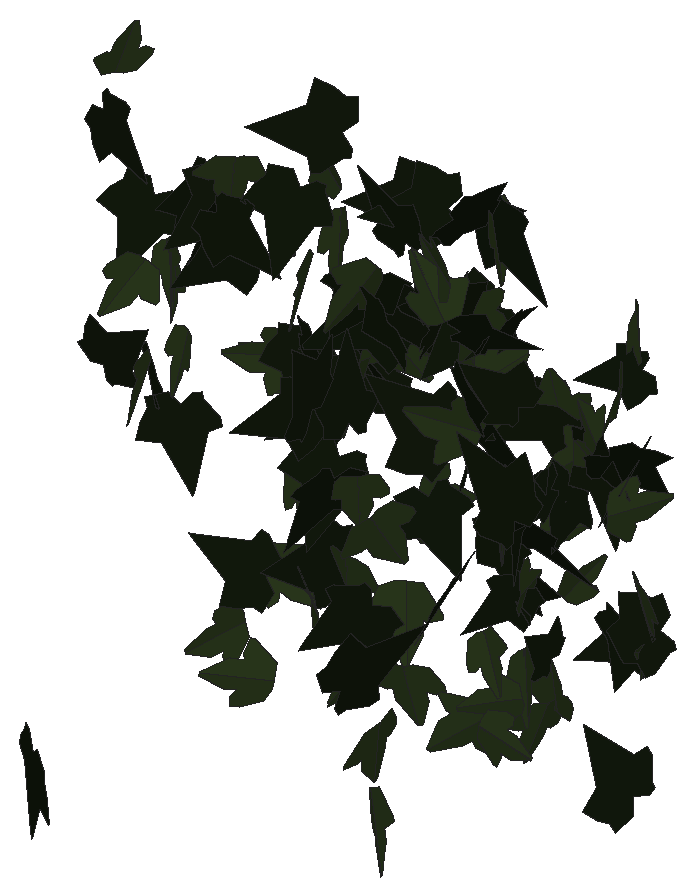
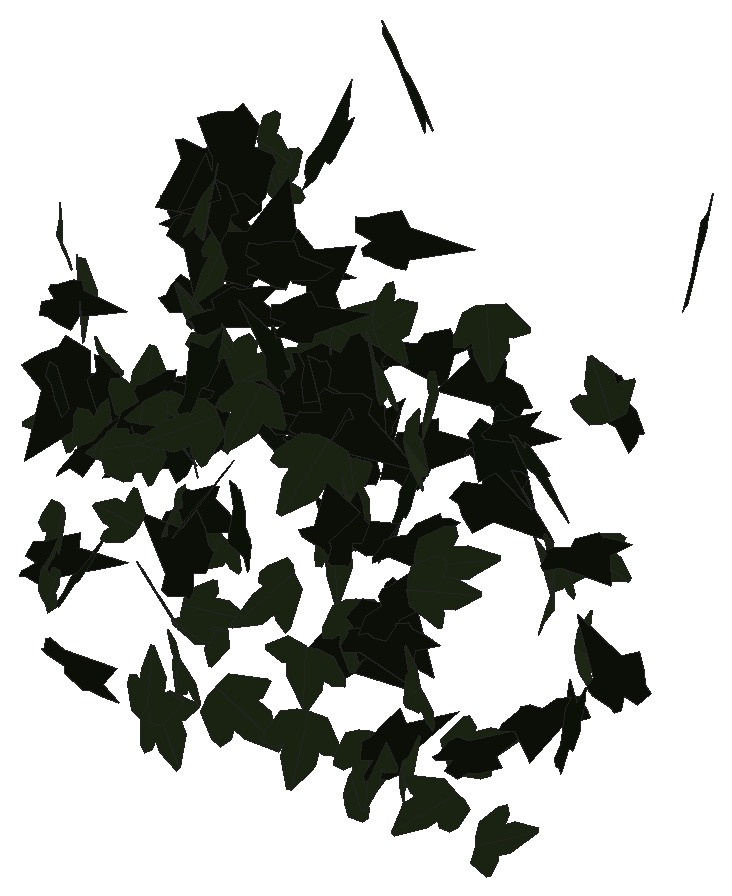
# SketchUp Ruby script. Lengths in inches.
U = 1.inch
M = Sketchup.active_model
def pt(a) = Geom::Point3d.new(a.map { |v| v * U })
def face(e, loops, mat)
  f = e.add_face(loops[0].map { |a| pt(a) })
  loops[1..].each { |l| e.add_face(l.map { |a| pt(a) }).erase! }
  f.material = f.back_material = mat if mat
  f
end
# faces: each face lists its corners as indices into pts; further lists are holes
def faces(e, pts, list, mat = nil) = list.each { |f| face(e, (f[0].is_a?(Array) ? f : [f]).map { |l| l.map { |i| pts[i] } }, mat) }
# xy, xz, yz: faces in a plane at the given z, y or x. An outline is a flat list of corners, or four numbers for a rectangle; further outlines are holes
def ring(l) = l.size == 4 ? [[l[0], l[1]], [l[2], l[1]], [l[2], l[3]], [l[0], l[3]]] : l.each_slice(2).to_a
def flat(e, list, mat, &to3) = list.each { |f| face(e, (f[0].is_a?(Array) ? f : [f]).map { |l| ring(l).map { |u, v| to3.(u, v) } }, mat) }
def xy(e, z, list, mat = nil) = flat(e, list, mat) { |x, y| [x, y, z] }
def xz(e, y, list, mat = nil) = flat(e, list, mat) { |x, z| [x, y, z] }
def yz(e, x, list, mat = nil) = flat(e, list, mat) { |y, z| [x, y, z] }
def lines(e, pts, list) = list.each { |a, b| e.add_line(pt(pts[a]), pt(pts[b])) }
# prism: a flat outline (further loops are holes) pulled along v
def prism(e, loops, v, mat = nil)
  f = face(e, loops, mat); d = Geom::Vector3d.new(v.map { |x| x * U })
  f.pushpull(f.normal.samedirection?(d) ? d.length : -d.length)
end
def box(e, o, s, mat = nil) = prism(e, [[o, [o[0] + s[0], o[1], o[2]], [o[0] + s[0], o[1] + s[1], o[2]], [o[0], o[1] + s[1], o[2]]]], [0, 0, s[2]], mat)
def at(x, y, z, deg = 0) = Geom::Transformation.translation(pt([x, y, z])) * Geom::Transformation.rotation(ORIGIN, Z_AXIS, deg.degrees)
def axes(o, x, y, z) = Geom::Transformation.new([*x, 0, *y, 0, *z, 0, *pt(o).to_a, 1])
def part(name) = M.definitions.add(name)
# library, detail: a bought-in or finely detailed component or shape, given as its bounding box
def library(name, o, s) = part(name).tap { |d| box(d.entities, o, s) }
def detail(e, o, s) = box(e.add_group.entities, o, s)
def put(e, d, t, mat = nil) = e.add_instance(d, t).tap { |i| i.material = mat if mat }
def group(e, t, mat = nil) = e.add_group.tap { |g| g.transformation = t; g.material = mat if mat }.entities
root = M.entities
M.materials.add("efeu1").color = [18, 25, 13]
M.materials.add("efeu2").color = [43, 57, 29]
c1 = part("ivyleaf_9")
p = [[1.54,2.16,1.25],[1.36,2.04,1.19],[-0.21,0.99,0.68],[-0.71,1.11,0.82],[-0.85,0.86,0.67],[-0.8,0.17,0.21],
  [-0.9,-0.01,0.1],[-0.67,-0.16,-0.02],[-0.08,-0.08,-0.05],[-0.03,-0.6,-0.4],[0.65,-0.88,-0.66],[0.83,-0.6,-0.49],
  [1.29,-0.42,-0.43],[1.8125,-0.07,-0.26],[1.21,0.44,0.15]]
faces(c1.entities,p,[[0,1,2,3,4,5,6,7,8,9,10,11,12,13,14]],"efeu1")
c2 = part("ivyleaf_10")
p = [[0,0.5,-0.03],[-0.0625,2.02,-0.43],[-0.19,2.01,-0.46],[-0.54,1.05,-0.29],[-0.52,0.625,-0.18],[-0.83,0.76,-0.28],
  [-1.16,0.64,-0.33],[-1.15,0.33,-0.24],[-0.77,-0.39,0.02],[-0.3,-0.51,0.16],[0.04,-0.48,0.23],[-0.02,2.01,-0.4375],
  [-0.06,2.01,-0.43],[0.04,-0.49,0.23],[0.67,-0.49,0.14],[1.38,0.36,-0.2],[1.375,0.51,-0.24],[0.81,0.65,-0.19],
  [0.62,0.59,-0.15],[0.6,1.09,-0.28],[0.5,1.23,-0.31]]
faces(c2.entities,p,[[0,1,2,3,4,5,6,7,8,9,10],[11,12,0,13,14,15,16,17,18,19,20]],"efeu2")
put(root,c1,axes([576.6875,99.81,193.13],[0.37598,-0.23293,-1.38227],[1.25923,-0.57264,0.43901],[-0.61586,-1.31306,0.05375]))
put(root,c2,axes([583.77,110.99,188.68],[-0.42455,1.04749,-0.55022],[0.21582,-0.5062,-1.13022],[-1.16335,-0.47618,-0.00888]))
put(root,c1,axes([580.52,111.29,204.13],[-0.34881,0.80332,1.20672],[-0.45266,1.11874,-0.8756],[-1.37717,-0.57118,-0.01783]))
put(root,c1,axes([579.57,114.39,190.66],[0.12861,0.13692,1.33146],[1.00054,0.87864,-0.187],[-0.88907,1.00862,-0.01785]))
put(root,c2,axes([579.82,116.01,188.12],[-0.00624,-1.2313,-0.24566],[0.00097,0.24566,-1.23131],[1.25556,-0.00631,-0.00027]))
put(root,c1,axes([578.77,117.87,204.16],[0.79532,-0.66978,-0.56365],[0.43288,-0.361,1.03978],[-0.76087,-0.90549,0.00238]))
put(root,c2,axes([579.15,116.83,196.28],[-0.58735,-0.9171,-0.59938],[0.3209,0.50625,-1.08906],[1.04755,-0.66929,-0.00245]))
put(root,c1,axes([585.18,117.21,198.54],[-0.07861,0.19519,1.39451],[-0.99968,0.97588,-0.19295],[-0.99166,-0.99925,0.08396]))
put(root,c1,axes([581.57,118.33,194.09],[-0.6526,0.81064,-0.47546],[0.30079,-0.36823,-1.04068],[-0.89035,-0.71858,-0.00308]))
put(root,c1,axes([579.63,119.36,196.36],[-0.04157,-0.87284,-0.66564],[0.05238,0.66378,-0.87368],[1.09644,-0.0648,0.0165]))
put(root,c2,axes([579.4,120.19,204.02],[0.9037,0.26235,0.6247],[-0.60418,-0.15932,0.94092],[0.30667,-1.08699,0.01286]))
put(root,c2,axes([570.34,120.92,184.91],[0.0741,0.27954,1.0388],[-0.499,-0.91353,0.28142],[0.95302,-0.50005,0.06658]))
put(root,c1,axes([580.01,120.97,200.04],[0.13894,-0.23607,0.99025],[0.46186,-0.87604,-0.27364],[0.90721,0.48214,-0.01235]))
put(root,c2,axes([579.59,120.0625,205.41],[-0.16108,0.12198,-1.11142],[-0.80563,0.76597,0.20083],[0.7753,0.82128,-0.02223]))
put(root,c1,axes([572.14,121.73,196.54],[-0.13488,-0.4355,-0.98711],[-0.03088,-0.99283,0.44225],[-1.07847,0.08289,0.11079]))
put(root,c2,axes([580.61,121.3125,189.78],[0.76357,-0.05982,0.61897],[0.61628,-0.05814,-0.76587],[0.08306,0.98122,-0.00765]))
put(root,c2,axes([580.89,121.37,186.2],[-0.24339,0.00696,-0.94198],[0.90391,-0.27215,-0.23557],[-0.26517,-0.93408,0.06162]))
put(root,c1,axes([579.82,121.11,202.6875],[0.72154,-0.01298,0.70616],[0.70553,0.05985,-0.71979],[-0.03261,1.00782,0.05184]))
put(root,c2,axes([581.09,122.14,187.29],[-0.10062,-0.13892,0.92067],[-0.59928,-0.69906,-0.17098],[0.7126,-0.60751,-0.01378]))
put(root,c2,axes([580.64,122.12,194.78],[-0.28531,0.51157,-0.73913],[0.34535,-0.65356,-0.58567],[-0.82991,-0.44785,0.01039]))
put(root,c1,axes([574.33,122.4,188.66],[0.0712,0.10786,-1.10788],[-0.49243,-0.99255,-0.12828],[-0.99827,0.4973,-0.01574]))
put(root,c2,axes([578.68,122.66,197.54],[-0.36943,-0.22943,-1.12963],[-0.96314,-0.59027,0.43487],[-0.63329,1.03156,-0.0024]))
put(root,c1,axes([581.09,122.76,191.55],[-0.03661,0.00225,-0.90716],[0.02991,-0.9074,-0.00345],[-0.90667,-0.03002,0.03652]))
put(root,c1,axes([577.67,122.625,202.2],[0.79036,0.26559,0.76895],[-0.7268,-0.25115,0.83377],[0.3655,-1.07372,-0.00482]))
put(root,c1,axes([573.625,122.07,196.45],[-0.43939,-0.68038,0.79048],[0.4057,0.67871,0.80969],[-0.96082,0.59772,-0.0196]))
put(root,c1,axes([581,122.63,199.39],[-0.03845,0.13449,0.9198],[-0.92952,0.00545,-0.03965],[-0.01112,-0.92059,0.13414]))
put(root,c1,axes([581.01,122.82,194.7],[-0.37558,-0.01683,-0.8276],[0.81422,-0.17129,-0.36603],[-0.14917,-0.89255,0.08584]))
put(root,c1,axes([577.45,122.69,196.76],[-1.01125,-0.48445,-0.67672],[-0.59369,-0.3264,1.12083],[-0.58325,1.17219,0.03242]))
put(root,c1,axes([581.4,122.35,194.54],[1.24264,-0.12436,0.23053],[0.22958,-0.02103,-1.24885],[0.12611,1.26367,0.00191]))
put(root,c1,axes([580.64,122.2,202.56],[0.05643,0.9385,0.17844],[0.00155,0.17866,-0.94015],[-0.95531,0.05572,0.00902]))
put(root,c2,axes([573.26,123.5,201.58],[-0.07924,-0.77106,0.88087],[-0.01064,-0.88238,-0.77333],[1.17062,-0.06022,0.0526]))
put(root,c2,axes([578.72,123.35,185.03],[-0.57796,-0.45111,0.95395],[-0.76465,-0.5705,-0.73306],[0.7272,-0.95842,-0.01265]))
put(root,c2,axes([579.44,122.43,202.56],[-0.10194,-0.82834,-0.8697],[0.27644,0.83321,-0.82599],[1.16881,-0.26931,0.11951]))
put(root,c2,axes([564.78,123.42,195.9375],[0.84954,-0.58492,0.13821],[0.11518,-0.07643,-1.03142],[0.58988,0.85731,0.00235]))
put(root,c1,axes([578.58,122.27,206.5],[0.5658,0.85095,0.73106],[0.39266,0.61678,-1.02181],[-1.0509,0.6886,0.01181]))
put(root,c1,axes([566.67,123.21,202.02],[0.0796,-0.21733,-1.11977],[0.93687,0.65277,-0.06009],[0.65068,-0.91329,0.22351]))
put(root,c1,axes([579.47,123.6,193.05],[0.53696,-1.07695,-0.0969],[-0.04223,0.08722,-1.20339],[1.08048,0.53862,0.00112]))
put(root,c2,axes([567.19,123.43,204.2],[-0.74535,-0.74022,0.08376],[-0.05925,-0.05921,-1.05046],[0.74258,-0.7477,0.00026]))
put(root,c2,axes([581.22,122.78,191.65],[-0.00272,-0.15871,-0.88095],[-0.07317,0.87805,-0.15796],[0.89214,0.07153,-0.01564]))
put(root,c1,axes([581.78,123.63,195.65],[-0.80952,0.29608,-0.1704],[0.15255,-0.07885,-0.8617],[-0.30566,-0.82349,0.02124]))
put(root,c2,axes([578.99,123.64,199.4],[0.73402,-0.27168,-0.86308],[0.83233,-0.23316,0.78126],[-0.35489,-1.10875,0.04719]))
put(root,c2,axes([566.47,124.34,184.18],[0.11187,0.15716,-1.04889],[-0.49494,-0.92508,-0.1914],[-0.93803,0.50685,-0.0241]))
put(root,c1,axes([578.38,123.94,197.02],[0.52187,-0.01064,-1.13102],[1.1276,0.10229,0.51933],[0.08845,-1.2414,0.05249]))
put(root,c2,axes([572.11,124.55,184.32],[0.00471,-0.14446,1.06579],[0.38185,-0.99615,-0.13671],[1.00547,0.37899,0.04692]))
put(root,c1,axes([567.87,124.27,186.92],[-0.52827,-0.84373,-0.40503],[-0.18535,-0.36157,0.99495],[-0.91738,0.55892,0.03221]))
put(root,c2,axes([562.1,124.5,193.34],[0.34739,-0.49754,0.88006],[0.50068,-0.72376,-0.60681],[0.87827,0.60939,-0.00217]))
put(root,c1,axes([579,123.96,205.91],[-0.17813,-0.08069,-1.29109],[1.20324,0.46823,-0.19528],[0.47502,-1.21631,0.01048]))
put(root,c1,axes([578.04,124.74,201.43],[-0.77449,-0.87377,0.45369],[-0.28368,-0.3547,-1.16741],[0.94278,-0.82453,0.02143]))
put(root,c2,axes([575.05,123.77,185.45],[-1.06568,-0.35712,-0.10063],[0.09572,0.03107,-1.12392],[0.35846,-1.06997,0.00095]))
put(root,c2,axes([574.7,123.97,188.46],[1.17891,0.23405,0.24291],[0.23853,0.04596,-1.20191],[-0.23851,1.20279,-0.00134]))
put(root,c1,axes([585.55,123.71,184.18],[-1.03675,-0.16771,-0.55972],[-0.55273,-0.08818,1.05022],[-0.18948,1.17488,-0.00107]))
put(root,c1,axes([571.08,124.34,191.92],[-0.17026,0.68314,-0.9242],[0.17731,-0.90749,-0.70345],[-1.13551,-0.24413,0.02873]))
put(root,c1,axes([560.51,124.23,203.73],[-0.00376,-0.1984,-1.09862],[1.06849,0.31772,-0.06103],[0.32351,-1.05168,0.18881]))
put(root,c1,axes([581.8,123.66,188.63],[-0.35075,0.51036,0.58361],[-0.33715,0.47641,-0.61924],[-0.69814,-0.48648,0.00583]))
put(root,c1,axes([572.98,124.18,201.08],[0.31311,0.62899,-0.95138],[-0.43056,-0.84839,-0.7026],[-1.05611,0.53235,0.00438]))
put(root,c2,axes([561.72,124.5625,197.375],[0.50217,0.5619,-0.68683],[-0.45573,-0.51386,-0.7536],[-0.76143,0.67813,-0.00193]))
put(root,c1,axes([571.125,124.59,206.5],[-0.7001,-0.05021,0.93375],[-0.92954,-0.08969,-0.70176],[0.10185,-1.16361,0.0138]))
put(root,c1,axes([581.73,124.95,195.07],[-0.07557,-0.90683,0.49811],[0.00475,-0.49973,-0.90906],[1.03461,-0.06394,0.04056]))
put(root,c2,axes([581.81,123.64,194],[-0.06949,-0.14341,-0.85498],[0.47056,0.71414,-0.15803],[0.72811,-0.47522,0.02053]))
put(root,c1,axes([574.51,124.16,203.42],[0.25263,-0.24003,1.001],[-0.7621,0.64925,0.34802],[-0.69197,-0.80268,-0.01784]))
put(root,c1,axes([569.05,124.85,203.19],[-0.62128,-0.96049,-0.15125],[0.0837,0.126,-1.14391],[0.96872,-0.62689,0.00183]))
put(root,c2,axes([578.71,124.44,205.7],[-0.32403,1.14319,-0.35051],[0.08306,-0.34075,-1.18816],[-1.19283,-0.33427,0.01248]))
put(root,c1,axes([575.75,124.0625,199.625],[-0.24948,0.97999,0.35571],[0.06059,-0.3515,1.0109],[1.04079,0.25537,0.02641]))
put(root,c1,axes([579.23,124.76,190.67],[0.30137,-0.30425,1.06123],[0.73438,-0.76612,-0.42819],[0.8243,0.79378,-0.00651]))
put(root,c2,axes([569.5,125,186],[-0.42874,0.09254,1.03856],[0.8937,-0.54581,0.41757],[0.53708,0.98209,0.13421]))
put(root,c2,axes([571.96,124.93,196.5625],[0.51208,-1.05709,0.37701],[0.17278,-0.33521,-1.17456],[1.10893,0.54037,0.00891]))
put(root,c2,axes([579.43,124.99,186.9],[0.81416,-0.35343,0.68704],[0.63444,-0.26378,-0.88753],[0.44093,1.03214,0.00844]))
put(root,c2,axes([584.4,124.36,200.44],[0.36155,-0.89247,-0.6503],[-0.22896,0.60881,-0.96283],[1.08026,0.42774,0.01358]))
put(root,c1,axes([572.9,125.22,199.24],[-0.02417,-0.06681,-1.27613],[-0.71896,-1.05448,0.06883],[-1.05644,0.71915,-0.01764]))
put(root,c2,axes([582.32,124.375,191.3],[-0.07325,-0.56841,0.60889],[0.06378,0.60561,0.57302],[-0.83052,0.09664,-0.0097]))
put(root,c1,axes([569.61,124.54,197.33],[0.73917,-0.3417,-0.62969],[-0.56379,0.28083,-0.8142],[0.44206,0.92953,0.01451]))
put(root,c1,axes([565.1875,125.74,201.1875],[-0.65175,-0.72254,0.59603],[-0.34064,-0.49356,-0.9708],[0.87252,-0.73241,0.06621]))
put(root,c1,axes([559.92,125.01,192.72],[-0.25218,0.04865,1.02424],[0.82065,-0.62281,0.23164],[0.61478,0.85133,0.11093]))
put(root,c2,axes([570.45,125.35,202.03],[0.88966,-0.48685,0.6537],[0.57213,-0.31622,-1.01416],[0.58053,1.05775,-0.00231]))
put(root,c2,axes([568.81,125.57,199.54],[0.53773,-0.67256,0.75229],[0.44877,-0.60411,-0.86086],[0.90381,0.7001,-0.02014]))
put(root,c1,axes([575.44,125.4375,204.45],[-0.77912,-0.09995,0.76812],[-0.7532,-0.15652,-0.78436],[0.18079,-1.08284,0.04247]))
put(root,c1,axes([573.13,124.91,200.1],[-0.00657,-0.0431,-1.13577],[0.96097,0.6063,-0.02857],[0.60694,-0.96042,0.03294]))
put(root,c2,axes([571.7,125.08,191.68],[-0.686,-0.72851,-0.02067],[0.02102,0.0086,-1.00062],[0.7285,-0.68626,0.00941]))
put(root,c1,axes([583.5,125.88,189.15],[0.03751,-0.82037,0.70868],[0.13206,-0.70037,-0.81773],[1.07601,0.11455,0.07565]))
put(root,c2,axes([580.0625,125.41,184.92],[-0.17895,-1.02248,0.25342],[-0.04918,-0.24866,-1.03801],[1.05227,-0.18551,-0.00542]))
put(root,c1,axes([584.5,125.375,196.99],[-0.6836,0.58659,-0.51199],[0.37107,-0.35352,-0.90047],[-0.68449,-0.77747,0.02316]))
put(root,c2,axes([567.77,125.72,195.43],[-0.01935,-0.00566,-1.13432],[-1.02381,-0.48838,0.0199],[-0.4884,1.02399,0.00322]))
put(root,c1,axes([580.33,126.1,197.55],[0.02923,-0.44999,-0.98319],[0.07057,-0.98066,0.45092],[-1.07897,-0.07633,0.00286]))
put(root,c1,axes([565.28,125.39,201.4],[-0.51176,0.84528,-0.61778],[0.32491,-0.52547,-0.98812],[-0.99529,-0.60617,-0.00492]))
put(root,c1,axes([568.75,125.79,196.17],[-0.26632,-1.07412,-0.0713],[0.02287,0.06779,-1.10662],[1.07624,-0.26724,0.00587]))
put(root,c1,axes([565.47,125.67,199.19],[0.07939,0.12689,-1.04983],[-0.50545,-0.92019,-0.14944],[-0.92886,0.51157,-0.00841]))
put(root,c2,axes([582.76,125.06,197.67],[0.37526,0.00151,0.76296],[-0.73429,0.23162,0.3607],[-0.2072,-0.8181,0.10353]))
put(root,c1,axes([569.77,126.25,187.21],[-0.30262,-0.34038,1.09723],[-0.73752,-0.81241,-0.45543],[0.88082,-0.79718,-0.00437]))
put(root,c1,axes([570.06,125.88,191.8],[-0.82605,-0.82852,-0.24431],[0.17565,0.16986,-1.16995],[0.84574,-0.8445,0.00436]))
put(root,c2,axes([584.25,124.6875,195.1875],[-0.02781,-0.01796,-1.04879],[0.63189,0.83714,-0.03109],[0.83726,-0.6324,-0.01137]))
put(root,c2,axes([583.97,125.87,202.53],[0.30666,-0.16322,0.86589],[0.74371,-0.44374,-0.34703],[0.47255,0.8043,-0.01575]))
put(root,c1,axes([584.77,126.15,189.66],[-0.68782,-0.42722,0.7466],[-0.64081,-0.38321,-0.80965],[0.57383,-0.94003,-0.00925]))
put(root,c1,axes([581.71,125.78,197.07],[0.1111,-0.09159,-1.13251],[1.10521,0.27269,0.08637],[0.26358,-1.10479,0.11521]))
put(root,c2,axes([580.34,125.71,185.34],[-1.03597,0.09791,0.07655],[0.07587,-0.01077,1.04059],[0.09844,1.03874,0.00357]))
put(root,c1,axes([562.72,125.89,191.375],[-0.22242,-0.97151,-0.4687],[0.11571,0.45431,-0.99659],[1.07244,-0.25051,0.01032]))
put(root,c1,axes([563.75,125.47,201.08],[-0.68215,0.69304,0.19759],[-0.13848,0.14094,-0.97244],[-0.70723,-0.69606,-0.00017]))
put(root,c2,axes([570.1,125.41,203.9],[-0.62813,0.36275,-0.8921],[-0.77022,0.45013,0.72535],[0.5781,0.99387,-0.00291]))
put(root,c1,axes([584.01,126.14,200.34],[-0.17639,-0.27745,-0.76457],[-0.35455,-0.67787,0.32778],[-0.73201,0.39519,0.02547]))
put(root,c2,axes([582.2,126.21,195.37],[-0.55821,-0.64537,-0.57934],[-0.35841,-0.45572,0.85299],[-0.78973,0.66299,0.02237]))
put(root,c2,axes([567.99,126.14,190.46],[0.6839,-0.27451,0.95007],[0.89755,-0.3127,-0.73644],[0.41521,1.12809,0.02706]))
put(root,c2,axes([580.35,126.05,197.31],[-0.77957,-0.70654,-0.25356],[-0.18552,-0.17288,1.0521],[-0.72738,0.80133,0.00341]))
put(root,c1,axes([583.58,125.1,196.97],[0.9835,0.74184,0.08712],[0.06641,0.05662,-1.2319],[-0.74398,0.98573,0.00519]))
put(root,c2,axes([567.54,126.02,202.0625],[-0.47563,0.829,-0.60657],[0.31204,-0.52025,-0.9557],[-0.97868,-0.56876,-0.00992]))
put(root,c2,axes([581.04,126.6,195.63],[-0.03992,-0.18331,1.05805],[0.00372,-1.0588,-0.1833],[1.07381,-0.00315,0.03997]))
put(root,c2,axes([561.89,126.0625,197.55],[0.73446,-0.27727,0.58688],[0.55834,-0.18206,-0.78476],[0.331,0.92234,0.02152]))
put(root,c2,axes([584.3,126.36,188.61],[-0.00797,-0.30077,-0.69642],[0.03601,-0.69582,0.3001],[-0.75774,-0.0299,0.02158]))
put(root,c1,axes([569.08,126.72,193.69],[0.11055,-0.41617,-1.00154],[0.24296,-0.97164,0.43056],[-1.057,-0.26687,-0.00578]))
put(root,c2,axes([578.22,125.41,197.16],[-0.30187,-0.26093,-1.05407],[0.91525,0.52759,-0.39272],[0.58434,-0.96116,0.07059]))
put(root,c2,axes([575.65,125.73,199.13],[-0.71364,-0.55909,-0.43768],[0.33722,0.27921,-0.9065],[0.62484,-0.78923,-0.01065]))
put(root,c2,axes([584.34,125.8125,191.3],[-0.81783,0.6453,0.02239],[-0.01865,0.01252,-1.04176],[-0.64542,-0.81804,0.00172]))
put(root,c1,axes([576.53,125.2,193.52],[0.00825,0.26816,1.04274],[-0.02697,1.04249,-0.26788],[-1.07633,-0.02406,0.01471]))
put(root,c2,axes([574.69,125.3,191.93],[-0.09313,-0.40606,-1.14802],[0.43692,1.06357,-0.41164],[1.13664,-0.44211,0.06417]))
put(root,c2,axes([572.74,125.82,197.94],[-0.86767,-0.60628,-0.60262],[0.50171,0.33403,-1.05844],[0.69211,-1.00221,0.01177]))
put(root,c1,axes([577.08,126.93,199.68],[0.21352,-0.70775,0.91452],[0.32357,-0.85627,-0.73821],[1.11021,0.38568,0.03926]))
put(root,c2,axes([559.66,126.23,204.65],[-0.35643,-0.88916,0.14535],[0.07062,0.12826,0.95778],[-0.89819,0.36293,0.01762]))
put(root,c1,axes([573.32,126.72,203.43],[-0.51517,-0.15717,0.83954],[-0.78689,-0.29395,-0.53789],[0.33217,-0.94012,0.02783]))
put(root,c1,axes([582.03,126.64,195.62],[0.13802,-1.12937,-0.07509],[-0.00795,0.07467,-1.13777],[1.13183,0.13824,0.00116]))
put(root,c2,axes([561.85,126.57,196.63],[-0.2669,0.69229,-0.65388],[0.18997,-0.62672,-0.74107],[-0.93313,-0.3256,0.03616]))
put(root,c1,axes([570.65,126.64,195.63],[0.29364,-0.36188,0.86209],[0.53112,-0.67909,-0.46597],[0.76946,0.60685,-0.00735]))
put(root,c1,axes([571.27,125.9,195.01],[-0.97896,-0.10643,0.69661],[0.69144,0.08506,0.9847],[-0.13601,1.1985,-0.00803]))
put(root,c2,axes([570.35,126.18,187.37],[-1.07987,-0.00447,0.20463],[-0.20459,-0.00803,-1.07986],[0.00589,-1.09906,0.00705]))
put(root,c2,axes([567.55,126.49,194.77],[-0.08527,0.03151,-1.04796],[-1.04609,-0.07288,0.08292],[-0.07012,1.0489,0.03725]))
put(root,c2,axes([567.12,125.88,186.28],[0.49146,0.48869,0.89138],[0.62523,0.63537,-0.69305],[-0.80154,0.79524,0.00595]))
put(root,c1,axes([560.5625,126.93,199],[-0.67448,-0.88403,-0.01548],[0.00936,0.01233,-1.11195],[0.88412,-0.67454,-0.00004]))
put(root,c1,axes([560.6,127.13,191.3125],[0.08778,-0.43073,1.07078],[0.23189,-1.0454,-0.43952],[1.13063,0.24785,0.00701]))
